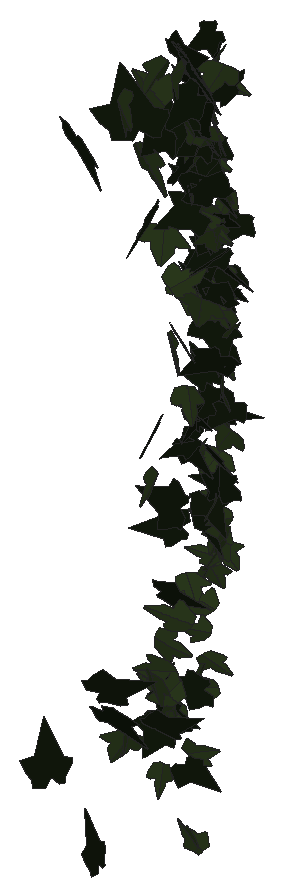
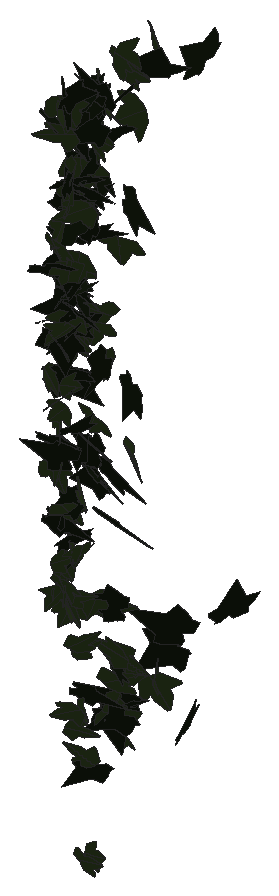
# SketchUp Ruby script. Lengths in inches.
U = 1.inch
M = Sketchup.active_model
def pt(a) = Geom::Point3d.new(a.map { |v| v * U })
def face(e, loops, mat)
  f = e.add_face(loops[0].map { |a| pt(a) })
  loops[1..].each { |l| e.add_face(l.map { |a| pt(a) }).erase! }
  f.material = f.back_material = mat if mat
  f
end
# faces: each face lists its corners as indices into pts; further lists are holes
def faces(e, pts, list, mat = nil) = list.each { |f| face(e, (f[0].is_a?(Array) ? f : [f]).map { |l| l.map { |i| pts[i] } }, mat) }
# xy, xz, yz: faces in a plane at the given z, y or x. An outline is a flat list of corners, or four numbers for a rectangle; further outlines are holes
def ring(l) = l.size == 4 ? [[l[0], l[1]], [l[2], l[1]], [l[2], l[3]], [l[0], l[3]]] : l.each_slice(2).to_a
def flat(e, list, mat, &to3) = list.each { |f| face(e, (f[0].is_a?(Array) ? f : [f]).map { |l| ring(l).map { |u, v| to3.(u, v) } }, mat) }
def xy(e, z, list, mat = nil) = flat(e, list, mat) { |x, y| [x, y, z] }
def xz(e, y, list, mat = nil) = flat(e, list, mat) { |x, z| [x, y, z] }
def yz(e, x, list, mat = nil) = flat(e, list, mat) { |y, z| [x, y, z] }
def lines(e, pts, list) = list.each { |a, b| e.add_line(pt(pts[a]), pt(pts[b])) }
# prism: a flat outline (further loops are holes) pulled along v
def prism(e, loops, v, mat = nil)
  f = face(e, loops, mat); d = Geom::Vector3d.new(v.map { |x| x * U })
  f.pushpull(f.normal.samedirection?(d) ? d.length : -d.length)
end
def box(e, o, s, mat = nil) = prism(e, [[o, [o[0] + s[0], o[1], o[2]], [o[0] + s[0], o[1] + s[1], o[2]], [o[0], o[1] + s[1], o[2]]]], [0, 0, s[2]], mat)
def at(x, y, z, deg = 0) = Geom::Transformation.translation(pt([x, y, z])) * Geom::Transformation.rotation(ORIGIN, Z_AXIS, deg.degrees)
def axes(o, x, y, z) = Geom::Transformation.new([*x, 0, *y, 0, *z, 0, *pt(o).to_a, 1])
def part(name) = M.definitions.add(name)
# library, detail: a bought-in or finely detailed component or shape, given as its bounding box
def library(name, o, s) = part(name).tap { |d| box(d.entities, o, s) }
def detail(e, o, s) = box(e.add_group.entities, o, s)
def put(e, d, t, mat = nil) = e.add_instance(d, t).tap { |i| i.material = mat if mat }
def group(e, t, mat = nil) = e.add_group.tap { |g| g.transformation = t; g.material = mat if mat }.entities
root = M.entities
M.materials.add("1026 AP 7946 SUNNY SIDE UP").color = [254, 231, 186]
M.materials.add("efeu1").color = [18, 25, 13]
M.materials.add("efeu2").color = [43, 57, 29]
c1 = part("ivyleaf_9")
p = [[1.54,2.16,1.25],[1.36,2.04,1.19],[-0.21,0.99,0.68],[-0.71,1.11,0.82],[-0.85,0.86,0.67],[-0.8,0.17,0.21],
  [-0.9,-0.01,0.1],[-0.67,-0.16,-0.02],[-0.08,-0.08,-0.05],[-0.03,-0.6,-0.4],[0.65,-0.88,-0.66],[0.83,-0.6,-0.49],
  [1.29,-0.42,-0.43],[1.8125,-0.07,-0.26],[1.21,0.44,0.15]]
faces(c1.entities,p,[[0,1,2,3,4,5,6,7,8,9,10,11,12,13,14]],"efeu1")
c2 = part("ivyleaf_10")
p = [[0,0.5,-0.03],[-0.0625,2.02,-0.43],[-0.19,2.01,-0.46],[-0.54,1.05,-0.29],[-0.52,0.625,-0.18],[-0.83,0.76,-0.28],
  [-1.16,0.64,-0.33],[-1.15,0.33,-0.24],[-0.77,-0.39,0.02],[-0.3,-0.51,0.16],[0.04,-0.48,0.23],[-0.02,2.01,-0.4375],
  [-0.06,2.01,-0.43],[0.04,-0.49,0.23],[0.67,-0.49,0.14],[1.38,0.36,-0.2],[1.375,0.51,-0.24],[0.81,0.65,-0.19],
  [0.62,0.59,-0.15],[0.6,1.09,-0.28],[0.5,1.23,-0.31]]
faces(c2.entities,p,[[0,1,2,3,4,5,6,7,8,9,10],[11,12,0,13,14,15,16,17,18,19,20]],"efeu2")
put(root,c1,axes([145.55,212.39,259.82],[-0.2417,-0.17789,0.08235],[0.06913,0.06887,0.24234],[-0.29944,0.15949,-0.01052]),"1026 AP 7946 SUNNY SIDE UP")
put(root,c1,axes([145.29,211.85,267.42],[0.36929,-0.13374,-0.1189],[-0.18067,0.02854,-0.27659],[0.20996,0.25979,-0.02888]),"1026 AP 7946 SUNNY SIDE UP")
put(root,c1,axes([145.63,211.78,258.76],[-0.35015,0.17835,-0.04553],[0.03425,-0.04493,-0.29337],[-0.28728,-0.22275,0.02052]),"1026 AP 7946 SUNNY SIDE UP")
put(root,c1,axes([145.48,212.2,265.41],[-0.4219,-0.09501,-0.08116],[0.14282,-0.0262,-0.28825],[0.13061,-0.27826,0.05302]),"1026 AP 7946 SUNNY SIDE UP")
put(root,c1,axes([145.18,211.96,266.89],[0.4492,-0.09852,-0.00584],[-0.02118,-0.02344,-0.31024],[0.15366,0.28476,-0.02569]),"1026 AP 7946 SUNNY SIDE UP")
put(root,c2,axes([145.36,211.38,261.08],[-0.17403,0.26419,-0.08669],[0.03586,-0.08325,-0.29536],[-0.43522,-0.1125,0.01033]),"1026 AP 7946 SUNNY SIDE UP")
put(root,c2,axes([145.61,212.3125,252.86],[0.08785,0.00972,-0.20061],[-0.28419,-0.07354,-0.05762],[-0.11521,0.18882,-0.01084]),"1026 AP 7946 SUNNY SIDE UP")
put(root,c2,axes([145.55,209.73,252.8],[-0.24204,-0.21864,0.12111],[-0.07602,-0.11075,-0.27516],[0.3838,-0.15982,0.02187]),"1026 AP 7946 SUNNY SIDE UP")
put(root,c2,axes([145.49,212.3,263.8],[-0.40147,0.03258,0.02484],[-0.04227,-0.02259,-0.26397],[-0.04746,-0.25544,0.02498]),"1026 AP 7946 SUNNY SIDE UP")
put(root,c1,axes([145.22,212.1875,264.4375],[0.05439,-0.06355,0.24415],[0.11964,-0.22515,-0.07484],[0.36738,0.08273,-0.01177]),"1026 AP 7946 SUNNY SIDE UP")
put(root,c1,axes([145.17,211.91,267.42],[0.29956,-0.21049,0.04665],[0.02846,-0.04619,-0.2922],[0.33775,0.19058,-0.01675]),"1026 AP 7946 SUNNY SIDE UP")
put(root,c2,axes([145.71,210.79,253.92],[0.18902,-0.02956,-0.26101],[-0.38851,0.05535,-0.12718],[0.0986,0.27476,-0.00077]),"1026 AP 7946 SUNNY SIDE UP")
put(root,c1,axes([145.16,211.86,267.3],[0.01344,0.02803,0.30266],[0.22726,-0.25646,0.01939],[0.4043,0.14323,-0.02096]),"1026 AP 7946 SUNNY SIDE UP")
put(root,c1,axes([145.48,210.64,264.41],[-0.29708,0.13089,-0.2728],[0.30093,-0.18634,-0.23599],[-0.35516,-0.26737,0.02823]),"1026 AP 7946 SUNNY SIDE UP")
put(root,c1,axes([145.39,211.54,261.15],[0.36282,-0.09319,-0.16858],[-0.24041,0.05693,-0.256],[0.17161,0.27678,-0.00223]),"1026 AP 7946 SUNNY SIDE UP")
put(root,c2,axes([145.66,211.65,249.64],[-0.09823,0.0529,-0.22012],[-0.22754,0.15791,0.08467],[0.26142,0.15732,-0.00902]),"1026 AP 7946 SUNNY SIDE UP")
put(root,c1,axes([145.28,211.08,252.73],[0.01828,-0.00044,-0.25547],[0.07317,0.24384,0.00323],[0.383,-0.04657,0.01157]),"1026 AP 7946 SUNNY SIDE UP")
put(root,c2,axes([145.34,211.91,262.14],[0.39344,0.11394,0.03422],[0.06152,-0.0076,-0.28229],[-0.17588,0.25221,-0.02219]),"1026 AP 7946 SUNNY SIDE UP")
put(root,c2,axes([145.4,212.27,257.1],[0.08136,0.24209,0.01501],[0.01232,0.01181,-0.2549],[-0.38102,0.05208,-0.00503]),"1026 AP 7946 SUNNY SIDE UP")
put(root,c2,axes([145.59,212.22,254.76],[0.08808,0.16496,0.17089],[-0.13098,-0.1443,0.17698],[0.34263,-0.09757,0.02373]),"1026 AP 7946 SUNNY SIDE UP")
put(root,c2,axes([145.37,211.06,263.7],[0.46921,0.06935,0.02199],[0.04037,-0.01819,-0.31478],[-0.10651,0.29858,-0.02244]),"1026 AP 7946 SUNNY SIDE UP")
put(root,c1,axes([145.41,212.47,263.09],[-0.13824,-0.17935,0.15344],[0.02433,-0.16432,-0.19408],[0.36679,-0.05669,0.0707]),"1026 AP 7946 SUNNY SIDE UP")
put(root,c2,axes([145.69,210.91,253.29],[0.2116,0.12253,0.21554],[-0.27951,-0.1117,0.18515],[0.25788,-0.22162,0.02382]),"1026 AP 7946 SUNNY SIDE UP")
put(root,c2,axes([145.5,212.65,260.99],[-0.01455,-0.07551,0.20971],[0.02257,-0.20394,-0.07829],[0.34128,0.01027,0.01412]),"1026 AP 7946 SUNNY SIDE UP")
put(root,c1,axes([145.5,212.55,267.6875],[-0.01823,-0.08128,-0.26056],[0.15738,-0.23536,0.07195],[-0.3862,-0.09207,0.04162]),"1026 AP 7946 SUNNY SIDE UP")
put(root,c2,axes([145.3,211.58,267.0625],[0.13444,-0.24522,-0.24839],[0.15482,-0.2191,0.26579],[-0.51652,-0.1295,0.01502]),"1026 AP 7946 SUNNY SIDE UP")
put(root,c1,axes([145.4,211.45,266.36],[-0.1312,-0.30662,-0.00538],[0.00855,0.00213,-0.32732],[0.48208,-0.08349,0.00434]),"1026 AP 7946 SUNNY SIDE UP")
put(root,c1,axes([145.83,211.02,257.17],[-0.38237,0.13769,0.10232],[-0.16679,0.01052,-0.28477],[-0.20751,-0.26217,0.04034]),"1026 AP 7946 SUNNY SIDE UP")
put(root,c1,axes([145.55,211.05,253.87],[-0.25367,0.08732,-0.16848],[0.19488,-0.11131,-0.18726],[-0.21773,-0.20136,0.02869]),"1026 AP 7946 SUNNY SIDE UP")
put(root,c2,axes([145.3,211.61,262.28],[0.2018,0.0805,-0.2575],[0.27629,0.1811,0.15381],[0.30776,-0.21535,0.03076]),"1026 AP 7946 SUNNY SIDE UP")
put(root,c1,axes([145.1875,208.5625,266.89],[0.18708,-0.31215,0.20885],[0.0901,-0.19682,-0.34499],[0.57983,0.1313,-0.01378]),"1026 AP 7946 SUNNY SIDE UP")
put(root,c2,axes([145.37,212.25,258.13],[0.08579,-0.16681,-0.18905],[0.10534,-0.16999,0.17964],[-0.37431,-0.08608,0.00723]),"1026 AP 7946 SUNNY SIDE UP")
put(root,c2,axes([145.48,212.47,266],[-0.21125,0.23176,-0.04361],[0.01575,-0.04458,-0.27588],[-0.37048,-0.13404,0.01314]),"1026 AP 7946 SUNNY SIDE UP")
put(root,c2,axes([145.7,212.32,255.89],[0.04408,0.06304,0.21087],[-0.21975,-0.15057,0.06673],[0.25449,-0.14094,0.0211]),"1026 AP 7946 SUNNY SIDE UP")
put(root,c2,axes([145.48,212.18,253.29],[0.1455,-0.15536,0.10986],[0.07196,-0.09773,-0.18662],[0.28824,0.10282,-0.00887]),"1026 AP 7946 SUNNY SIDE UP")
put(root,c1,axes([145.41,212.36,262.6],[-0.23077,-0.10195,-0.17683],[0.30198,-0.01623,-0.15986],[0.08285,-0.22481,0.09014]),"1026 AP 7946 SUNNY SIDE UP")
put(root,c2,axes([145.73,211.8,249.5],[0.1689,0.0074,0.19952],[-0.3033,0.0252,0.10939],[-0.02906,-0.21999,0.01794]),"1026 AP 7946 SUNNY SIDE UP")
put(root,c2,axes([145.8,211.32,266.09],[-0.10322,0.06287,-0.30733],[-0.30174,0.22908,0.09447],[0.37322,0.20259,-0.00862]),"1026 AP 7946 SUNNY SIDE UP")
put(root,c1,axes([145.41,212.26,262.29],[0.14152,-0.20974,-0.13012],[-0.08474,0.113,-0.23442],[0.37455,0.10481,-0.00387]),"1026 AP 7946 SUNNY SIDE UP")
put(root,c2,axes([145.53,210.62,253.76],[-0.34774,0.14432,-0.02754],[0.01632,-0.03432,-0.27122],[-0.23045,-0.2202,0.02235]),"1026 AP 7946 SUNNY SIDE UP")
put(root,c1,axes([145.22,209.32,253.93],[0.06452,0.0024,0.30973],[0.47008,0.03182,-0.04211],[-0.05008,0.30175,0.00377]),"1026 AP 7946 SUNNY SIDE UP")
put(root,c2,axes([145.34,212.27,264.98],[-0.19897,-0.10029,-0.22667],[0.32408,0.08393,-0.16145],[0.19728,-0.23902,0.0366]),"1026 AP 7946 SUNNY SIDE UP")
put(root,c2,axes([145.51,210.87,252.5],[-0.33429,-0.11712,0.05378],[0.06022,0.03981,0.24974],[-0.19287,0.21543,-0.01524]),"1026 AP 7946 SUNNY SIDE UP")
put(root,c2,axes([145.23,211.27,254.23],[0.00276,-0.0345,-0.28863],[0.38016,-0.14406,0.019],[-0.22852,-0.24007,0.02813]),"1026 AP 7946 SUNNY SIDE UP")
put(root,c1,axes([145.26,211.94,259.22],[0.21829,-0.03801,-0.20076],[0.31009,0.0012,0.14466],[-0.03316,-0.23909,0.03121]),"1026 AP 7946 SUNNY SIDE UP")
put(root,c2,axes([145.89,210.34,267.28],[0.20731,0.05181,0.33387],[-0.50181,0.10047,0.1179],[-0.11848,-0.33486,0.08485]),"1026 AP 7946 SUNNY SIDE UP")
put(root,c2,axes([145.58,211.3,252.83],[0.09106,0.14606,-0.17674],[-0.10333,-0.15938,-0.16279],[-0.33992,0.08758,0.00214]),"1026 AP 7946 SUNNY SIDE UP")
put(root,c1,axes([145.65,210.98,252.55],[0.07335,0.21884,-0.10336],[-0.03027,-0.09975,-0.23109],[-0.37816,0.05043,-0.00155]),"1026 AP 7946 SUNNY SIDE UP")
put(root,c2,axes([145.54,212.45,263.64],[-0.33209,-0.1807,-0.01814],[0.1056,-0.05421,-0.27304],[0.26506,-0.2048,0.08605]),"1026 AP 7946 SUNNY SIDE UP")
put(root,c2,axes([145.42,211.83,264.62],[-0.08076,0.09067,-0.26684],[0.13757,-0.24491,-0.10741],[-0.4098,-0.10009,0.01653]),"1026 AP 7946 SUNNY SIDE UP")
put(root,c1,axes([145.23,211.3,255.33],[0.21947,-0.02606,0.20892],[0.29639,-0.07919,-0.14449],[0.12516,0.23323,-0.02418]),"1026 AP 7946 SUNNY SIDE UP")
put(root,c2,axes([145.625,212.52,258.07],[0.30018,0.07871,-0.1115],[-0.14194,-0.06451,-0.21186],[-0.15612,0.20999,-0.02178]),"1026 AP 7946 SUNNY SIDE UP")
put(root,c1,axes([145.88,211.96,259.59],[-0.29542,0.1646,0.10414],[-0.14045,0.04955,-0.2562],[-0.26845,-0.20706,0.01943]),"1026 AP 7946 SUNNY SIDE UP")
put(root,c1,axes([145.73,211.73,264.01],[-0.2667,-0.14723,0.20055],[-0.2066,-0.14591,-0.23148],[0.32468,-0.21378,0.01744]),"1026 AP 7946 SUNNY SIDE UP")
put(root,c1,axes([145.52,212.21,265.02],[-0.21023,-0.234,0.09801],[0.06052,-0.12663,-0.26221],[0.39335,-0.10558,0.09273]),"1026 AP 7946 SUNNY SIDE UP")
put(root,c1,axes([145.6,210.71,252.64],[-0.17899,-0.21314,0.08128],[-0.04391,-0.07582,-0.24913],[0.35533,-0.11673,0.01016]),"1026 AP 7946 SUNNY SIDE UP")
put(root,c1,axes([145.48,212.63,265.53],[-0.01513,-0.03387,0.25783],[0.01058,-0.2506,-0.03611],[0.39728,0.00538,0.01078]),"1026 AP 7946 SUNNY SIDE UP")
put(root,c2,axes([145.67,211.96,265.75],[-0.36858,-0.17786,0.02257],[-0.00545,-0.03322,-0.30229],[0.28193,-0.23317,0.02366]),"1026 AP 7946 SUNNY SIDE UP")
put(root,c2,axes([145.63,212.37,255.73],[0.08654,-0.2303,0.05352],[-0.00268,-0.05507,-0.24382],[0.37167,0.05322,-0.01422]),"1026 AP 7946 SUNNY SIDE UP")
put(root,c2,axes([145.64,210.84,252.87],[-0.00114,0.12825,0.22424],[-0.11374,0.2077,-0.12553],[-0.37959,-0.06262,0.03694]),"1026 AP 7946 SUNNY SIDE UP")
put(root,c1,axes([145.37,209.27,253.52],[0.48102,0.01022,0.01833],[0.02932,-0.02958,-0.31397],[-0.01328,0.30499,-0.02927]),"1026 AP 7946 SUNNY SIDE UP")
put(root,c1,axes([145.35,211.82,258.53],[-0.01436,-0.03386,-0.24678],[0.36962,0.05461,-0.01688],[0.08864,-0.23322,0.03041]),"1026 AP 7946 SUNNY SIDE UP")
put(root,c2,axes([145.67,212.375,265.36],[-0.31515,0.19876,0.05779],[-0.09005,0.01998,-0.28947],[-0.31151,-0.20686,0.02522]),"1026 AP 7946 SUNNY SIDE UP")
put(root,c2,axes([145.4375,212.46,253.39],[-0.18865,-0.03637,-0.16776],[0.25976,0.0005,-0.12565],[0.03459,-0.2021,0.02866]),"1026 AP 7946 SUNNY SIDE UP")
put(root,c1,axes([145.63,212.24,263.65],[0.27015,0.17331,-0.09418],[-0.08647,-0.07541,-0.25149],[-0.29648,0.17992,-0.01247]),"1026 AP 7946 SUNNY SIDE UP")
put(root,c1,axes([145.64,212.06,259.3],[-0.10794,0.08385,-0.24753],[0.19428,-0.20714,-0.11183],[-0.35064,-0.14059,0.01424]),"1026 AP 7946 SUNNY SIDE UP")
put(root,c2,axes([145.66,212.41,261.86],[-0.30891,-0.15471,-0.0061],[0.02562,-0.01256,-0.25687],[0.24205,-0.19612,0.0194]),"1026 AP 7946 SUNNY SIDE UP")
put(root,c2,axes([145.52,211.71,255.54],[0.21794,0.18522,0.03926],[0.05207,0.02142,-0.23779],[-0.29241,0.14186,-0.01308]),"1026 AP 7946 SUNNY SIDE UP")
put(root,c2,axes([145.65,210.39,258.46],[0.24532,-0.28208,0.00402],[-0.01071,-0.01006,-0.33196],[0.4435,0.15579,-0.01024]),"1026 AP 7946 SUNNY SIDE UP")
put(root,c2,axes([145.62,210.6875,267.74],[0.00769,-0.22685,0.26838],[0.0821,-0.25836,-0.23314],[0.53848,0.04263,0.03172]),"1026 AP 7946 SUNNY SIDE UP")
put(root,c1,axes([145.52,212.54,267.09],[0.02037,0.14102,0.2557],[-0.05802,-0.24474,0.14427],[0.444,-0.03845,0.00712]),"1026 AP 7946 SUNNY SIDE UP")
put(root,c1,axes([145.84,209.7,266.9],[-0.5435,-0.14826,0.1424],[0.17539,0.09101,0.38609],[-0.26721,0.36129,-0.03622]),"1026 AP 7946 SUNNY SIDE UP")
put(root,c1,axes([145.5625,212.27,263.28],[0.2149,-0.14268,-0.16624],[-0.17079,0.11827,-0.20283],[0.29138,0.17456,0.00372]),"1026 AP 7946 SUNNY SIDE UP")
put(root,c2,axes([145.58,212.62,267.1],[-0.03183,-0.09358,-0.27493],[0.01612,-0.26709,0.09431],[-0.44359,-0.00299,0.02315]),"1026 AP 7946 SUNNY SIDE UP")
put(root,c1,axes([145.72,207.0625,253.2],[-0.26003,-0.23615,0.2395],[0.2604,0.16787,0.29631],[-0.45303,0.23203,0.03285]),"1026 AP 7946 SUNNY SIDE UP")
put(root,c2,axes([145.63,212.57,256.35],[0.342,-0.07148,-0.0107],[-0.02411,-0.01481,-0.23515],[0.1109,0.21722,-0.01813]),"1026 AP 7946 SUNNY SIDE UP")
put(root,c1,axes([145.72,212.5,261.97],[0.24225,0.13261,-0.14493],[-0.17709,-0.08582,-0.20979],[-0.24814,0.19072,0.00824]),"1026 AP 7946 SUNNY SIDE UP")
put(root,c2,axes([145.93,211.02,255.0625],[0.0755,0.06442,0.27364],[-0.34664,-0.14968,0.07769],[0.25312,-0.2242,0.02476]),"1026 AP 7946 SUNNY SIDE UP")
put(root,c1,axes([145.81,211.12,265.23],[0.01433,0.20811,0.25584],[-0.01733,0.24732,-0.21267],[-0.50777,-0.00257,0.01448]),"1026 AP 7946 SUNNY SIDE UP")
put(root,c2,axes([145.64,212.42,255.84],[0.19584,-0.19669,0.05126],[0.03236,-0.04716,-0.23999],[0.31782,0.12601,-0.00715]),"1026 AP 7946 SUNNY SIDE UP")
put(root,c2,axes([145.72,212.35,256.19],[-0.13322,0.16898,0.11096],[-0.11172,0.08291,-0.19281],[-0.29376,-0.10817,0.023]),"1026 AP 7946 SUNNY SIDE UP")
put(root,c1,axes([145.46,212.38,258.22],[0.35312,-0.09304,0.0026],[-0.00822,-0.02057,-0.24961],[0.14615,0.22365,-0.02033]),"1026 AP 7946 SUNNY SIDE UP")
put(root,c2,axes([145.5,211.68,259.8],[0.37034,-0.06099,0.14437],[0.20384,-0.05783,-0.2501],[0.12822,0.26807,-0.01939]),"1026 AP 7946 SUNNY SIDE UP")
put(root,c1,axes([146,211.54,253.28],[-0.12192,-0.08905,-0.22785],[-0.28928,-0.12476,0.11773],[-0.2373,0.19784,-0.02646]),"1026 AP 7946 SUNNY SIDE UP")
put(root,c2,axes([145.62,212.4,262.41],[-0.31767,-0.10025,-0.10293],[0.17215,-0.00184,-0.22746],[0.14005,-0.22512,0.04611]),"1026 AP 7946 SUNNY SIDE UP")
put(root,c1,axes([145.52,212.14,256.83],[0.15918,-0.23995,-0.02195],[-0.00836,0.0194,-0.26816],[0.3785,0.10134,0.00331]),"1026 AP 7946 SUNNY SIDE UP")
put(root,c2,axes([145.53,209.69,252.84],[0.01212,0.00877,0.30236],[0.27664,-0.23514,0.0011],[0.36955,0.17573,-0.01074]),"1026 AP 7946 SUNNY SIDE UP")
put(root,c1,axes([145.6875,212.2,265.48],[-0.21813,-0.26092,-0.00125],[0.01624,-0.00579,-0.30422],[0.40996,-0.13861,0.01139]),"1026 AP 7946 SUNNY SIDE UP")
put(root,c2,axes([145.8,211.86,254.4],[0.01832,0.08532,0.2137],[-0.05343,-0.20416,0.08748],[0.34791,-0.03585,0.00218]),"1026 AP 7946 SUNNY SIDE UP")
put(root,c2,axes([145.8125,212.125,257.24],[0.07825,-0.21953,-0.15056],[-0.05361,0.14084,-0.23107],[0.41011,0.0603,-0.00148]),"1026 AP 7946 SUNNY SIDE UP")
put(root,c1,axes([145.91,210,259.67],[-0.13102,0.08596,-0.32172],[-0.34716,0.22156,0.12462],[0.37368,0.23598,0.00297]),"1026 AP 7946 SUNNY SIDE UP")
put(root,c1,axes([145.91,212.17,263.05],[-0.42516,-0.00418,-0.02186],[0.03379,-0.02442,-0.27757],[0.00353,-0.27012,0.02383]),"1026 AP 7946 SUNNY SIDE UP")
put(root,c1,axes([145.46,212.39,264.4],[0.16191,-0.24591,0.10779],[0.14018,-0.07564,-0.27036],[0.39707,0.12698,0.0515]),"1026 AP 7946 SUNNY SIDE UP")
put(root,c2,axes([145.72,212.26,255.6],[-0.24329,-0.13334,-0.0737],[0.10423,0.03105,-0.20936],[0.21327,-0.16729,0.01824]),"1026 AP 7946 SUNNY SIDE UP")
put(root,c1,axes([145.52,211.7,267.41],[0.30821,-0.24627,-0.02221],[-0.0478,0.00151,-0.32339],[0.38557,0.19704,-0.02234]),"1026 AP 7946 SUNNY SIDE UP")
put(root,c1,axes([145.49,212,265.67],[0.09594,-0.1501,0.2312],[0.16339,-0.20025,-0.16762],[0.39305,0.11989,0.01324]),"1026 AP 7946 SUNNY SIDE UP")
put(root,c1,axes([145.625,212.17,257.25],[0.04253,-0.23223,-0.12315],[-0.01741,0.11773,-0.24016],[0.40939,0.02914,0.00258]),"1026 AP 7946 SUNNY SIDE UP")
put(root,c1,axes([146.03,211.96,261.96],[0.07969,0.02489,0.28584],[-0.38588,0.13715,0.03433],[-0.20681,-0.24631,0.04609]),"1026 AP 7946 SUNNY SIDE UP")
put(root,c2,axes([145.5625,212.66,261.77],[0.01209,-0.09582,-0.21472],[0.22075,-0.16231,0.08147],[-0.28429,-0.13011,0.05413]),"1026 AP 7946 SUNNY SIDE UP")
put(root,c2,axes([145.88,211.7,262],[-0.43442,-0.05672,0.05317],[-0.07185,-0.03471,-0.28967],[0.09727,-0.27897,0.02351]),"1026 AP 7946 SUNNY SIDE UP")
put(root,c1,axes([145.79,212.3,257.5],[-0.00166,0.05534,0.24425],[-0.19481,-0.20386,0.04733],[0.329,-0.12044,0.02925]),"1026 AP 7946 SUNNY SIDE UP")
put(root,c2,axes([145.68,212.54,260.34],[-0.27146,0.07614,-0.10763],[0.1384,-0.05941,-0.19399],[-0.14963,-0.19308,0.01584]),"1026 AP 7946 SUNNY SIDE UP")
put(root,c1,axes([146.08,212.36,257.63],[-0.11507,-0.01617,-0.23702],[-0.32313,-0.1048,0.07434],[-0.16433,0.2174,0.01978]),"1026 AP 7946 SUNNY SIDE UP")
put(root,c1,axes([146.19,210.54,257.96],[-0.23862,-0.0265,-0.31453],[-0.48165,0.01393,0.15576],[0.00114,0.34053,-0.02884]),"1026 AP 7946 SUNNY SIDE UP")
put(root,c1,axes([145.8,211.78,265.71],[-0.16423,-0.16001,0.24658],[-0.10312,-0.23567,-0.19244],[0.44203,-0.11443,0.04672]),"1026 AP 7946 SUNNY SIDE UP")
put(root,c2,axes([145.64,212.45,262.19],[0.13412,0.19385,0.15566],[0.11951,0.13007,-0.21694],[-0.3664,0.11338,-0.01378]),"1026 AP 7946 SUNNY SIDE UP")
put(root,c1,axes([145.72,212.65,260.57],[-0.06673,-0.22086,0.11861],[-0.02073,-0.11591,-0.23223],[0.39201,-0.04373,0.00791]),"1026 AP 7946 SUNNY SIDE UP")
put(root,c2,axes([145.82,212.49,258.98],[-0.21016,0.18317,0.01971],[-0.04071,0.00343,-0.23276],[-0.28653,-0.13483,0.01861]),"1026 AP 7946 SUNNY SIDE UP")
put(root,c2,axes([145.84,212.51,256.71],[-0.01222,0.01375,0.21831],[-0.00589,-0.21195,0.01279],[0.33374,-0.00324,0.00822]),"1026 AP 7946 SUNNY SIDE UP")
put(root,c2,axes([145.87,211.66,265.64],[-0.08924,-0.26221,0.12978],[0.00533,-0.13044,-0.27564],[0.4584,-0.04953,0.02847]),"1026 AP 7946 SUNNY SIDE UP")
put(root,c1,axes([145.6875,212.35,261.16],[-0.19045,-0.19288,-0.14068],[0.1763,0.08682,-0.23012],[0.326,-0.15964,0.04226]),"1026 AP 7946 SUNNY SIDE UP")
put(root,c2,axes([145.55,212.125,263.55],[-0.16979,0.0101,-0.25186],[0.36052,-0.08932,-0.10863],[-0.13461,-0.25195,0.02675]),"1026 AP 7946 SUNNY SIDE UP")
put(root,c2,axes([145.89,212.38,256.12],[0.01226,0.15457,-0.19059],[-0.13015,-0.17303,-0.15282],[-0.35715,0.06836,0.04915]),"1026 AP 7946 SUNNY SIDE UP")
put(root,c1,axes([146.08,211.73,264.52],[0.08068,0.04459,0.30638],[-0.46112,-0.05821,0.06083],[0.10289,-0.29587,0.03237]),"1026 AP 7946 SUNNY SIDE UP")
put(root,c2,axes([145.83,212.54,264.12],[0.37602,-0.13774,0.015],[0.00746,-0.02244,-0.28389],[0.2178,0.23858,-0.01617]),"1026 AP 7946 SUNNY SIDE UP")
put(root,c1,axes([146.0625,211.78,262.99],[-0.09742,0.30194,0.01377],[-0.03603,0.00717,-0.31676],[-0.47376,-0.06263,0.02126]),"1026 AP 7946 SUNNY SIDE UP")
put(root,c1,axes([145.72,211.84,266.03],[-0.08899,0.13388,0.27972],[0.07381,-0.26823,0.14517],[0.46918,0.06759,0.03022]),"1026 AP 7946 SUNNY SIDE UP")
put(root,c2,axes([145.61,212.51,266.74],[-0.15665,-0.07159,-0.23924],[0.37891,-0.00005,-0.10667],[0.04437,-0.25232,0.0663]),"1026 AP 7946 SUNNY SIDE UP")
put(root,c2,axes([145.63,209.5,267.39],[-0.04471,-0.00648,-0.40417],[0.2365,-0.36345,-0.00717],[-0.56978,-0.15035,0.02874]),"1026 AP 7946 SUNNY SIDE UP")
put(root,c2,axes([146.17,212.05,261.78],[-0.25585,0.02451,0.23137],[-0.34265,-0.08946,-0.1532],[0.09292,-0.26239,0.07212]),"1026 AP 7946 SUNNY SIDE UP")
put(root,c2,axes([146,212.15,267.17],[-0.32493,-0.17042,0.12329],[-0.07006,-0.12983,-0.26833],[0.32076,-0.201,0.06628]),"1026 AP 7946 SUNNY SIDE UP")
put(root,c1,axes([145.61,210.63,252.66],[0.03534,-0.00632,0.26382],[0.40207,0.01661,-0.02259],[-0.02516,0.25657,0.00947]),"1026 AP 7946 SUNNY SIDE UP")
put(root,c1,axes([146.09,211.96,260.73],[0.00165,0.08788,-0.26631],[-0.12683,-0.24739,-0.08826],[-0.41093,0.07671,0.02617]),"1026 AP 7946 SUNNY SIDE UP")
put(root,c2,axes([145.93,212.22,256.59],[-0.07679,-0.22801,0.10648],[0.02863,-0.10956,-0.23779],[0.39344,-0.03653,0.03809]),"1026 AP 7946 SUNNY SIDE UP")
put(root,c2,axes([146.08,212.34,258.79],[-0.34312,0.01598,0.11605],[-0.17875,-0.03412,-0.22225],[0.00253,-0.24316,0.03735]),"1026 AP 7946 SUNNY SIDE UP")
put(root,c2,axes([145.91,212.35,264.43],[-0.26905,0.21976,-0.00388],[-0.00867,-0.01064,-0.28677],[-0.34554,-0.17085,0.01021]),"1026 AP 7946 SUNNY SIDE UP")
put(root,c2,axes([145.82,212.43,256.02],[0.14061,0.19084,0.12206],[0.05099,0.11404,-0.21577],[-0.3486,0.09366,0.01767]),"1026 AP 7946 SUNNY SIDE UP")
put(root,c1,axes([145.77,211.36,251.52],[0.01735,-0.08489,-0.2411],[0.02903,0.23341,-0.08514],[0.38966,-0.01361,0.01708]),"1026 AP 7946 SUNNY SIDE UP")
put(root,c1,axes([145.82,212.56,262.42],[-0.1431,-0.24584,0.05196],[0.08134,-0.07228,-0.26004],[0.3866,-0.07579,0.07394]),"1026 AP 7946 SUNNY SIDE UP")
put(root,c2,axes([145.95,211.98,263.5],[-0.15858,-0.24711,-0.07575],[0.0519,0.06441,-0.27451],[0.40143,-0.10594,0.00557]),"1026 AP 7946 SUNNY SIDE UP")
put(root,c1,axes([146.02,208.18,250.84],[-0.06867,-0.25105,0.23002],[0.1315,0.21141,0.26132],[-0.5132,0.08777,0.03618]),"1026 AP 7946 SUNNY SIDE UP")
put(root,c1,axes([145.65,212.36,262.625],[0.32064,-0.10082,0.10371],[0.1274,-0.06374,-0.23387],[0.18506,0.21857,-0.0187]),"1026 AP 7946 SUNNY SIDE UP")
put(root,c1,axes([145.91,210.44,266.54],[-0.12753,-0.21898,0.26318],[-0.11458,-0.24642,-0.24171],[0.51804,-0.10841,0.01133]),"1026 AP 7946 SUNNY SIDE UP")
put(root,c1,axes([145.78,212.46,261.82],[0.05272,-0.21549,0.10689],[0.02766,-0.10351,-0.22527],[0.37589,0.03784,0.00158]),"1026 AP 7946 SUNNY SIDE UP")
put(root,c1,axes([145.99,212.68,263.6],[-0.29814,-0.18246,0.00992],[0.00665,-0.01974,-0.27063],[0.28732,-0.18888,0.01655]),"1026 AP 7946 SUNNY SIDE UP")
put(root,c2,axes([145.85,210.4375,251.87],[0.33,-0.12099,0.1118],[0.12553,-0.07893,-0.24858],[0.22344,0.22303,-0.02547]),"1026 AP 7946 SUNNY SIDE UP")
put(root,c2,axes([145.78,211.56,251.73],[-0.19138,-0.03157,0.18558],[0.25651,0.07956,0.12825],[-0.13063,0.20249,-0.02006]),"1026 AP 7946 SUNNY SIDE UP")
put(root,c2,axes([146.11,212.11,259.85],[-0.19081,0.15402,0.1826],[-0.20385,0.12124,-0.20025],[-0.30662,-0.17645,0.01949]),"1026 AP 7946 SUNNY SIDE UP")
put(root,c1,axes([145.66,212.43,259.14],[0.1376,-0.02304,0.2345],[0.34858,-0.05227,-0.0935],[0.08976,0.23833,0.00364]),"1026 AP 7946 SUNNY SIDE UP")
put(root,c1,axes([146.08,212.41,259.49],[-0.37199,-0.07671,-0.02546],[0.04768,-0.01516,-0.25514],[0.11719,-0.23733,0.02299]),"1026 AP 7946 SUNNY SIDE UP")
put(root,c1,axes([146.23,212.27,266.83],[-0.33822,0.21146,-0.01445],[-0.00412,-0.02433,-0.31026],[-0.33334,-0.21426,0.01849]),"1026 AP 7946 SUNNY SIDE UP")
put(root,c2,axes([145.76,210.01,266.125],[-0.341,0.19485,-0.26297],[0.27239,-0.18996,-0.30081],[-0.42683,-0.2769,0.01812]),"1026 AP 7946 SUNNY SIDE UP")
put(root,c1,axes([146.125,211.16,267.04],[-0.47623,0.08144,-0.14386],[0.19541,-0.07388,-0.32143],[-0.16355,-0.32542,0.03485]),"1026 AP 7946 SUNNY SIDE UP")
put(root,c2,axes([146.01,212.58,261.07],[0.057,-0.23442,0.07996],[0.02515,-0.0774,-0.24479],[0.38813,0.03944,0.00412]),"1026 AP 7946 SUNNY SIDE UP")
